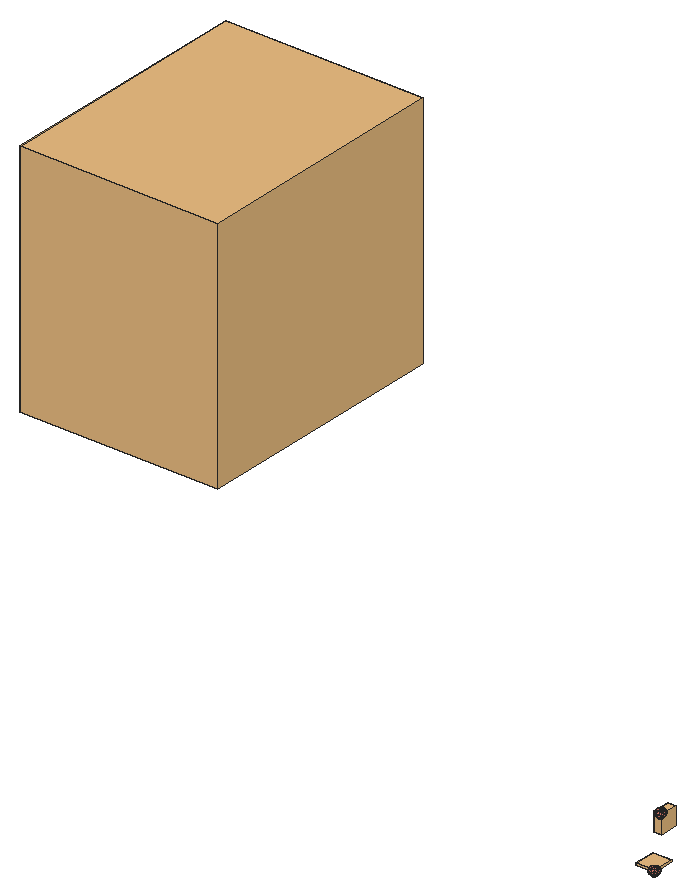
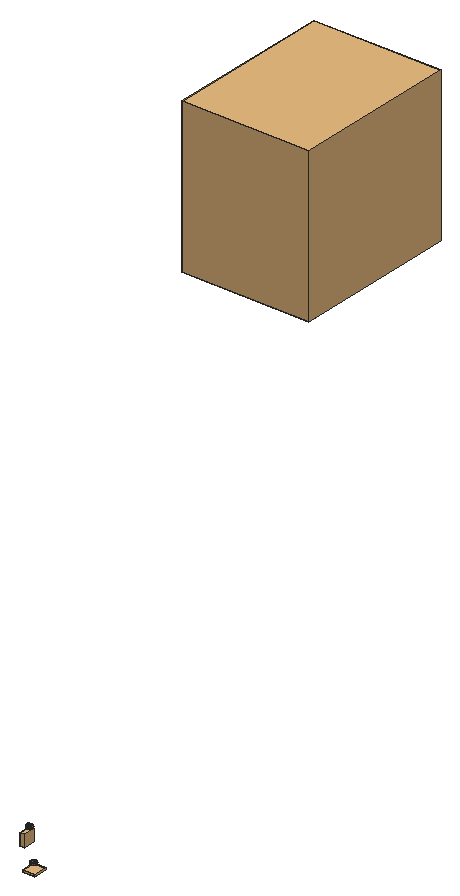
# SketchUp Ruby script. Lengths in inches.
U = 1.inch
M = Sketchup.active_model
def pt(a) = Geom::Point3d.new(a.map { |v| v * U })
def face(e, loops, mat)
  f = e.add_face(loops[0].map { |a| pt(a) })
  loops[1..].each { |l| e.add_face(l.map { |a| pt(a) }).erase! }
  f.material = f.back_material = mat if mat
  f
end
# faces: each face lists its corners as indices into pts; further lists are holes
def faces(e, pts, list, mat = nil) = list.each { |f| face(e, (f[0].is_a?(Array) ? f : [f]).map { |l| l.map { |i| pts[i] } }, mat) }
# xy, xz, yz: faces in a plane at the given z, y or x. An outline is a flat list of corners, or four numbers for a rectangle; further outlines are holes
def ring(l) = l.size == 4 ? [[l[0], l[1]], [l[2], l[1]], [l[2], l[3]], [l[0], l[3]]] : l.each_slice(2).to_a
def flat(e, list, mat, &to3) = list.each { |f| face(e, (f[0].is_a?(Array) ? f : [f]).map { |l| ring(l).map { |u, v| to3.(u, v) } }, mat) }
def xy(e, z, list, mat = nil) = flat(e, list, mat) { |x, y| [x, y, z] }
def xz(e, y, list, mat = nil) = flat(e, list, mat) { |x, z| [x, y, z] }
def yz(e, x, list, mat = nil) = flat(e, list, mat) { |y, z| [x, y, z] }
def lines(e, pts, list) = list.each { |a, b| e.add_line(pt(pts[a]), pt(pts[b])) }
# prism: a flat outline (further loops are holes) pulled along v
def prism(e, loops, v, mat = nil)
  f = face(e, loops, mat); d = Geom::Vector3d.new(v.map { |x| x * U })
  f.pushpull(f.normal.samedirection?(d) ? d.length : -d.length)
end
def box(e, o, s, mat = nil) = prism(e, [[o, [o[0] + s[0], o[1], o[2]], [o[0] + s[0], o[1] + s[1], o[2]], [o[0], o[1] + s[1], o[2]]]], [0, 0, s[2]], mat)
def at(x, y, z, deg = 0) = Geom::Transformation.translation(pt([x, y, z])) * Geom::Transformation.rotation(ORIGIN, Z_AXIS, deg.degrees)
def axes(o, x, y, z) = Geom::Transformation.new([*x, 0, *y, 0, *z, 0, *pt(o).to_a, 1])
def part(name) = M.definitions.add(name)
# library, detail: a bought-in or finely detailed component or shape, given as its bounding box
def library(name, o, s) = part(name).tap { |d| box(d.entities, o, s) }
def detail(e, o, s) = box(e.add_group.entities, o, s)
def put(e, d, t, mat = nil) = e.add_instance(d, t).tap { |i| i.material = mat if mat }
def group(e, t, mat = nil) = e.add_group.tap { |g| g.transformation = t; g.material = mat if mat }.entities
root = M.entities
M.materials.add("green").color = [174, 139, 102]
M.materials.add("vio").color = [206, 114, 100]
c1 = library("Untitled",[0,0,0],[7.78,10.125,9.38])
c2 = part("3DGeom~190_Defintion")
p = [[103.5625,-60.76,-498.22],[-159.65,90.28,-476.73],[101.5,52.12,-500],[335.44,0,-389.29],[150.07,151.03,-458.14],[-75.51,261.6,-404.23],
  [155.72,-157.36,-453.28],[-156.07,-105.24,-473.65],[-378.01,104.24,-325.73],[-280.86,302.07,-242.01],[-280.86,302.07,-242.01],[-65.73,-272.55,-395.81],
  [-373.88,-121.52,-322.17],[236.28,209.48,-383.86],[73.81,362.83,-275.57],[73.81,362.83,-275.57],[243.99,-211.79,-377.22],[-75.51,261.6,-404.23],
  [-280.86,302.07,-242.01],[-108.44,418.95,-93.44],[-75.51,261.6,-404.23],[73.81,362.83,-275.57],[87.16,-366.83,-264.07],[-269.57,-314.71,-232.28],
  [-65.73,-272.55,-395.81],[87.16,-366.83,-264.07],[-269.57,-314.71,-232.28],[344.72,-209.48,-290.42],[430.93,-151.03,-216.13],[344.72,-209.48,-290.42],
  [335.44,0,-389.29],[479.51,-52.12,-174.27],[335.44,0,-389.29],[477.44,60.76,-176.05],[335.44,0,-389.29],[337.02,211.79,-297.06],
  [425.29,157.36,-221],[335.44,0,-389.29],[337.02,211.79,-297.06],[335.44,0,-389.29],[236.28,209.48,-383.86],[248.29,366.83,-125.23],
  [236.28,209.48,-383.86],[248.29,366.83,-125.23],[337.02,211.79,-297.06],[344.72,-209.48,-290.42],[87.16,-366.83,-264.07],[243.99,-211.79,-377.22],
  [-373.88,-121.52,-322.17],[-495.09,90.28,-87.4375],[-378.01,104.24,-325.73],[-378.01,104.24,-325.73],[-410.95,261.6,-14.9375],[-378.01,104.24,-325.73],
  [-410.95,261.6,-14.9375],[-280.86,302.07,-242.01],[-269.57,-314.71,-232.28],[-491.51,-105.24,-84.36],[-373.88,-121.52,-322.17],[-373.88,-121.52,-322.17],
  [401.18,272.55,6.52],[248.29,366.83,-125.23],[344.72,-209.48,-290.42],[261.64,-362.83,-113.72],[87.16,-366.83,-264.07],[261.64,-362.83,-113.72],
  [344.72,-209.48,-290.42],[93.03,423.58,80.16],[248.29,366.83,-125.23],[87.16,-366.83,-264.07],[-93.03,-423.58,-80.16],[-269.57,-314.71,-232.28],
  [87.16,-366.83,-264.07],[-410.95,261.6,-14.9375],[-261.64,362.83,113.72],[-401.18,-272.55,-6.52],[-269.57,-314.71,-232.28],[-269.57,-314.71,-232.28],
  [-401.18,-272.55,-6.52],[491.51,105.23,84.36],[410.95,-261.6,14.9375],[261.64,-362.83,-113.72],[495.09,-90.28,87.44],[248.29,366.83,-125.23],
  [269.57,314.71,232.28],[401.18,272.55,6.52],[248.29,366.83,-125.23],[269.57,314.71,232.28],[108.44,-418.95,93.44],[410.95,-261.6,14.9375],
  [-87.16,366.83,264.07],[-479.51,52.12,174.27],[-430.93,151.03,216.13],[-410.95,261.6,-14.9375],[-477.44,-60.76,176.05],[-248.29,-366.83,125.23],
  [-401.18,-272.55,-6.52],[-410.95,261.6,-14.9375],[-344.72,209.48,290.42],[-410.95,261.6,-14.9375],[-344.72,209.48,290.42],[-261.64,362.83,113.72],
  [-248.29,-366.83,125.23],[-425.29,-157.36,221],[373.88,121.52,322.17],[269.57,314.71,232.28],[410.95,-261.6,14.9375],[280.86,-302.07,242.01],
  [280.86,-302.07,242.01],[65.73,272.55,395.81],[65.73,272.55,395.81],[269.57,314.71,232.28],[378.01,-104.24,325.73],[280.86,-302.07,242.01],
  [-73.81,-362.83,275.57],[-344.72,209.48,290.42],[-243.99,211.79,377.22],[-243.99,211.79,377.22],[-248.29,-366.83,125.23],[-337.02,-211.79,297.06],
  [-337.02,-211.79,297.06],[-335.44,0,389.29],[-344.72,209.48,290.42],[269.57,314.71,232.28],[65.73,272.55,395.81],[156.07,105.24,473.65],
  [269.57,314.71,232.28],[373.88,121.52,322.17],[75.51,-261.6,404.23],[378.01,-104.24,325.73],[75.51,-261.6,404.23],[280.86,-302.07,242.01],
  [-87.16,366.83,264.07],[-243.99,211.79,377.22],[-155.72,157.36,453.28],[-87.16,366.83,264.07],[-236.28,-209.48,383.86],[-337.02,-211.79,297.06],
  [75.51,-261.6,404.23],[-236.28,-209.48,383.86],[-73.81,-362.83,275.57],[-344.72,209.48,290.42],[-335.44,0,389.29],[-337.02,-211.79,297.06],
  [-236.28,-209.48,383.86],[-335.44,0,389.29],[373.88,121.52,322.17],[159.65,-90.28,476.73],[378.01,-104.24,325.73],[373.88,121.52,322.17],
  [378.01,-104.24,325.73],[75.51,-261.6,404.23],[-335.44,0,389.29],[75.51,-261.6,404.23],[-150.07,-151.03,458.14],[-236.28,-209.48,383.86],
  [-236.28,-209.48,383.86],[-335.44,0,389.29],[-101.5,-52.12,500],[-335.44,0,389.29],[-103.5625,60.76,498.22],[-335.44,0,389.29],
  [-335.44,0,389.29],[75.51,-261.6,404.23]]
faces(c2.entities,p,[[0,1,2],[0,2,3],[2,4,3],[2,1,5],[2,5,4],[6,7,0],[6,0,3],[0,7,1],
  [7,8,1],[1,8,9],[1,10,5],[11,12,7],[6,11,7],[7,12,8],[4,13,3],[4,5,14],
  [4,15,13],[16,11,6],[16,6,3],[17,18,19],[20,19,21],[22,23,24],[16,25,11],[11,26,12],
  [27,16,3],[28,29,30],[31,28,32],[33,31,34],[13,35,3],[36,33,37],[38,36,39],[40,21,41],
  [42,43,44],[45,46,47],[48,49,50],[51,49,52],[53,54,55],[56,57,58],[59,57,49],[38,60,36],
  [38,61,60],[62,63,64],[28,65,66],[21,19,67],[21,67,68],[69,70,71],[63,70,72],[18,73,74],
  [18,74,19],[70,75,76],[77,78,57],[36,79,33],[36,60,79],[28,80,81],[31,80,28],[33,79,82],
  [33,82,31],[31,82,80],[83,84,85],[86,67,87],[63,88,70],[89,88,63],[19,74,90],[19,90,67],
  [57,91,49],[49,91,92],[49,92,93],[78,94,57],[57,94,91],[70,95,96],[88,95,70],[97,92,98],
  [99,100,101],[102,103,78],[78,103,94],[60,104,79],[60,105,104],[106,107,88],[82,108,80],[67,90,109],
  [67,110,111],[79,104,112],[79,112,82],[82,112,113],[88,114,95],[107,114,88],[74,115,116],[74,117,90],
  [118,119,103],[114,120,95],[91,94,121],[92,91,121],[94,103,121],[122,92,121],[103,119,121],[123,124,125],
  [126,125,127],[107,128,114],[129,130,131],[132,133,134],[135,134,124],[114,136,137],[138,139,140],[133,141,142],
  [143,144,145],[146,147,148],[149,125,147],[150,147,151],[134,133,152],[153,154,155],[156,154,157],[154,158,159],
  [158,160,161],[160,134,162],[124,134,160],[124,160,125],[147,154,163],[147,158,154],[125,158,147],[125,160,158]],"vio")
c3 = part("3DGeom~191_Defintion")
p = [[58.83,-275.51,-375.83],[-159.55,-167.25,-431.01],[-6.51,0,-500],[191.37,-130.67,-435.58],[-202.64,130.67,-430.45],[148.28,167.25,-435.02],
  [-68.59,275.51,-374.17],[261.44,-309.94,-219.95],[261.44,-309.94,-219.95],[337.97,-226.32,-254.44],[337.97,-226.32,-254.44],[325.42,14.17,-379.3],
  [325.42,14.17,-379.3],[325.42,14.17,-379.3],[263.34,289.68,-253.47],[31.05,381.54,-216.95],[31.05,381.54,-216.95],[263.34,289.68,-253.47],
  [-36.6875,-381.54,-216.07],[-269.84,-289.68,-246.53],[-36.6875,-381.54,-216.07],[-335.18,-14.17,-370.7],[-344.47,226.32,-245.5625],[-267.08,309.94,-213.07],
  [-267.08,309.94,-213.07],[337.97,-226.32,-254.44],[325.42,14.17,-379.3],[415.36,-142.7,-221.95],[415.36,-142.7,-221.95],[325.42,14.17,-379.3],
  [425.06,120.2,-222.07],[325.42,14.17,-379.3],[263.34,289.68,-253.47],[425.06,120.2,-222.07],[206.3,-371.16,-127.71],[-36.6875,-381.54,-216.07],
  [58.83,-275.51,-375.83],[206.3,-371.16,-127.71],[58.83,-275.51,-375.83],[261.44,-309.94,-219.95],[-68.59,275.51,-374.17],[-267.08,309.94,-213.07],
  [-209.55,371.16,-122.29],[-68.59,275.51,-374.17],[31.05,381.54,-216.95],[-430.69,-120.2,-210.9375],[-430.69,-120.2,-210.9375],[-420.99,142.7,-211.06],
  [-335.18,-14.17,-370.7],[-420.99,142.7,-211.06],[261.44,-309.94,-219.95],[337.97,-226.32,-254.44],[394.01,-261.34,-5.125],[394.01,-261.34,-5.125],
  [263.34,289.68,-253.47],[307.83,334.49,-4.01],[263.34,289.68,-253.47],[69.59,420.35,-0.9],[263.34,289.68,-253.47],[307.83,334.49,-4.01],
  [-69.59,-420.35,0.9],[-307.83,-334.49,4.01],[-269.84,-289.68,-246.53],[-269.84,-289.68,-246.53],[-307.83,-334.49,4.01],[-430.69,-120.2,-210.9375],
  [-269.84,-289.68,-246.53],[-344.47,226.32,-245.5625],[-420.99,142.7,-211.06],[-394.01,261.34,5.125],[-267.08,309.94,-213.07],[-344.47,226.32,-245.5625],
  [472.89,-81.48,-131.17],[463.59,159.01,-6.03],[394.01,-261.34,-5.125],[206.3,-371.16,-127.71],[394.01,-261.34,-5.125],[-187.3,393.57,2.4375],
  [187.3,-393.57,-2.4375],[206.3,-371.16,-127.71],[-209.55,371.16,-122.29],[-267.08,309.94,-213.07],[-430.69,-120.2,-210.9375],[-476.14,81.48,-118.83],
  [-420.99,142.7,-211.06],[-420.99,142.7,-211.06],[-307.83,-334.49,4.01],[-463.59,-159.01,6.03],[-430.69,-120.2,-210.9375],[-430.69,-120.2,-210.9375],
  [495.13,-59.08,-6.44],[394.01,-261.34,-5.125],[206.3,-371.16,-127.71],[394.01,-261.34,-5.125],[-394.01,261.34,5.125],[-495.13,59.08,6.44],
  [476.14,-81.48,118.83],[394.01,-261.34,-5.125],[430.69,120.2,210.9375],[269.84,289.68,246.53],[269.84,289.68,246.53],[209.55,-371.16,122.29],
  [267.08,-309.94,213.07],[209.55,-371.16,122.29],[394.01,-261.34,-5.125],[344.47,-226.32,245.5625],[394.01,-261.34,-5.125],[420.99,-142.7,211.06],
  [394.01,-261.34,-5.125],[394.01,-261.34,-5.125],[307.83,334.49,-4.01],[36.6875,381.54,216.07],[269.84,289.68,246.53],[307.83,334.49,-4.01],
  [36.6875,381.54,216.07],[-206.3,371.16,127.71],[36.6875,381.54,216.07],[-31.05,-381.54,216.95],[-394.01,261.34,5.125],[-263.34,-289.68,253.47],
  [-263.34,-289.68,253.47],[-307.83,-334.49,4.01],[-472.89,81.48,131.17],[-415.36,142.7,221.95],[-337.97,226.32,254.44],[-337.97,226.32,254.44],
  [-261.44,309.94,219.95],[-261.44,309.94,219.95],[-206.3,371.16,127.71],[-263.34,-289.68,253.47],[-425.06,-120.2,222.07],[335.18,14.17,370.7],
  [335.18,14.17,370.7],[267.08,-309.94,213.07],[36.6875,381.54,216.07],[-261.44,309.94,219.95],[-325.42,-14.17,379.3],[-325.42,-14.17,379.3],
  [430.69,120.2,210.9375],[159.55,167.25,431.01],[335.18,14.17,370.7],[430.69,120.2,210.9375],[269.84,289.68,246.53],[420.99,-142.7,211.06],
  [202.64,-130.67,430.45],[344.47,-226.32,245.5625],[420.99,-142.7,211.06],[267.08,-309.94,213.07],[68.59,-275.51,374.17],[344.47,-226.32,245.5625],
  [68.59,-275.51,374.17],[267.08,-309.94,213.07],[36.6875,381.54,216.07],[-261.44,309.94,219.95],[-58.83,275.51,375.83],[36.6875,381.54,216.07],
  [-58.83,275.51,375.83],[68.59,-275.51,374.17],[-263.34,-289.68,253.47],[-31.05,-381.54,216.95],[-261.44,309.94,219.95],[-337.97,226.32,254.44],
  [-191.37,130.67,435.58],[-415.36,142.7,221.95],[-325.42,-14.17,379.3],[-415.36,142.7,221.95],[-148.28,-167.25,435.02],[-425.06,-120.2,222.07],
  [-263.34,-289.68,253.47],[-425.06,-120.2,222.07],[344.47,-226.32,245.5625],[68.59,-275.51,374.17],[68.59,-275.51,374.17],[-263.34,-289.68,253.47],
  [6.51,0,500],[68.59,-275.51,374.17]]
faces(c3.entities,p,[[0,1,2],[0,2,3],[1,4,2],[3,2,5],[2,4,6],[2,6,5],[7,0,3],[8,3,9],
  [10,3,11],[3,5,12],[13,5,14],[5,6,15],[5,16,17],[18,19,1],[20,1,0],[19,21,1],
  [1,21,4],[21,22,4],[4,22,23],[4,24,6],[25,26,27],[28,29,30],[31,32,33],[34,35,36],
  [37,38,39],[40,41,42],[43,42,44],[19,45,21],[46,47,48],[21,49,22],[50,51,52],[51,28,53],
  [30,54,55],[56,44,57],[58,57,59],[60,61,62],[60,63,35],[64,65,66],[67,68,69],[70,71,69],
  [28,30,72],[72,30,73],[30,55,73],[28,72,74],[75,50,76],[44,42,77],[44,77,57],[78,60,35],
  [78,35,79],[80,81,69],[82,83,84],[85,83,69],[86,87,88],[87,83,89],[72,90,91],[72,73,90],
  [78,92,93],[77,42,94],[87,95,83],[83,95,69],[90,96,97],[90,98,96],[90,73,98],[73,99,98],
  [73,55,100],[101,78,93],[102,103,104],[105,102,106],[107,105,108],[96,107,109],[110,111,112],[113,57,114],
  [101,60,78],[57,77,115],[57,115,116],[117,61,60],[101,117,60],[115,77,118],[117,119,61],[120,87,121],
  [95,122,69],[122,123,69],[123,124,69],[125,126,69],[127,128,69],[129,130,87],[130,95,87],[130,122,95],
  [96,131,107],[96,98,132],[133,117,101],[134,115,135],[136,122,130],[137,123,122],[138,139,140],[141,142,139],
  [143,144,145],[146,140,144],[147,148,117],[149,150,151],[152,153,154],[142,155,156],[157,158,159],[156,160,161],
  [162,163,164],[162,161,165],[166,167,168],[166,164,169],[170,144,171],[142,156,139],[172,166,173],[156,161,162],
  [140,174,144],[140,139,174],[144,166,175],[139,156,162],[174,164,166],[174,162,164],[144,174,166],[139,162,174]],"vio")
c4 = library("3DGeom~11_Defintion",[-500,-49.41,-434.02],[1000,98.82,868.04])
c5 = part("3DGeom~12_Defintion")
p = [[-473.91,-42.88,-428.57],[-493.27,-23.3125,-425.27],[-480.23,-29.84,-434.02],[-473.91,-42.88,-428.57],[-480.23,-29.84,-434.02],[-475.54,-36.36,-433.07],
  [-493.27,-23.3125,-425.27],[-486.72,-25.0625,-431.16],[-480.23,-29.84,-434.02],[-480.63,-49.41,-414.38],[-493.27,-23.3125,-425.27],[-473.91,-42.88,-428.57],
  [-480.63,-49.41,-414.38],[-473.91,-42.88,-428.57],[-475.77,-47.66,-421.73],[-493.68,-42.88,-405.63],[-493.27,-23.3125,-425.27],[-480.63,-49.41,-414.38],
  [-500,-29.84,-411.07],[-493.27,-23.3125,-425.27],[-493.68,-42.88,-405.63],[-493.27,-23.3125,-425.27],[-498.13,-25.0625,-417.92],[-493.68,-42.88,-405.63],
  [-480.63,-49.41,-414.38],[-487.1875,-47.66,-408.48],[-493.68,-42.88,-405.63],[-498.37,-36.36,-406.58],[489.39,27.6,421.47],[498.07,5.37,408.95],
  [500,12.78,407.52],[489.39,27.6,421.47],[500,12.78,407.52],[498.875,20.1875,409.65],[489.39,27.6,421.47],[493.59,-0.05,413.55],
  [498.07,5.37,408.95],[489.39,27.6,421.47],[498.875,20.1875,409.65],[494.99,25.61,414.75],[489.39,27.6,421.47],[487.78,-2.04,420.08],
  [493.59,-0.05,413.55],[489.39,27.6,421.47],[482.18,-0.05,426.79],[487.78,-2.04,420.08],[489.39,27.6,421.47],[478.3,5.37,431.9],
  [482.18,-0.05,426.79],[489.39,27.6,421.47],[477.17,12.78,434.02],[478.3,5.37,431.9],[489.39,27.6,421.47],[479.1,20.1875,432.59],
  [477.17,12.78,434.02],[489.39,27.6,421.47],[483.58,25.61,428],[479.1,20.1875,432.59]]
faces(c5.entities,p,[[0,1,2],[3,4,5],[6,7,8],[9,10,11],[12,13,14],[15,16,17],[18,19,20],[21,18,22],
  [23,24,25],[18,26,27],[28,29,30],[31,32,33],[34,35,36],[37,38,39],[40,41,42],[43,44,45],
  [46,47,48],[49,50,51],[52,53,54],[55,56,57]],"green")
c6 = library("3DGeom~13_Defintion",[-468.3,-500,-197.66],[936.6,1000,395.32])
c7 = part("3DGeom~14_Defintion")
p = [[-455.16,-492.22,-183.4],[-446.73,-497.16,-180.84],[-439.77,-500,-173.64],[-436.83,-497.09,-153.74],[-455.16,-492.22,-183.4],[-439.77,-500,-173.64],
  [-449.28,-486.4,-143.61],[-455.16,-492.22,-183.4],[-436.83,-497.09,-153.74],[-467.61,-481.53,-173.27],[-455.16,-492.22,-183.4],[-464.67,-478.62,-153.38],
  [-455.16,-492.22,-183.4],[-467.61,-481.53,-173.27],[-462.81,-486.5,-180.63],[-464.67,-478.62,-153.38],[-455.16,-492.22,-183.4],[-449.28,-486.4,-143.61],
  [-436.83,-497.09,-153.74],[-439.77,-500,-173.64],[-436.15,-499.97,-163.72],[-467.61,-481.53,-173.27],[-464.67,-478.62,-153.38],[-468.3,-478.65,-163.3],
  [-449.28,-486.4,-143.61],[-436.83,-497.09,-153.74],[-441.64,-492.12,-146.38],[-464.67,-478.62,-153.38],[-449.28,-486.4,-143.61],[-457.71,-481.46,-146.17],
  [456.2,493.0625,159.13],[456.82,479.16,194.97],[464.16,476.9375,187.85],[456.2,493.0625,159.13],[464.16,476.9375,187.85],[468.3,477.81,178.18],
  [456.2,493.0625,159.13],[468.3,477.81,178.18],[468.13,481.53,168.58],[456.2,493.0625,159.13],[448.25,483.875,197.66],[456.82,479.16,194.97],
  [456.2,493.0625,159.13],[468.13,481.53,168.58],[463.7,487.12,161.6],[456.2,493.0625,159.13],[440.74,489.82,195.18],[448.25,483.875,197.66],
  [456.2,493.0625,159.13],[436.3125,495.41,188.21],[440.74,489.82,195.18],[456.2,493.0625,159.13],[436.15,499.13,178.6],[436.3125,495.41,188.21],
  [456.2,493.0625,159.13],[440.29,500,168.94],[436.15,499.13,178.6],[456.2,493.0625,159.13],[447.63,497.78,161.8125],[440.29,500,168.94]]
faces(c7.entities,p,[[0,1,2],[3,4,5],[6,7,8],[9,10,11],[12,13,14],[15,16,17],[18,19,20],[21,22,23],
  [24,25,26],[27,28,29],[30,31,32],[33,34,35],[36,37,38],[39,40,41],[42,43,44],[45,46,47],
  [48,49,50],[51,52,53],[54,55,56],[57,58,59]],"green")
put(root,c1,at(12.99,12.95,61.14))
g1 = group(root,at(15.3125,38.42,26.21))
put(g1,c2,axes([2.9,-0.75,9.71],[0,0.00038,0],[0,0,-0.00038],[-0.00038,0,0]),"vio")
g2 = group(root,at(15.3125,38.42,26.21))
put(g2,c3,axes([3.03,-0.6,11.73],[0,0.00039,0],[0,0,-0.00039],[-0.00039,0,0]),"vio")
g3 = group(root,at(15.3125,38.42,26.21))
put(g3,c4,axes([2.51,-0.3,9.67],[0,0.00085,0],[0,0,-0.00085],[-0.00085,0,0]),"green")
put(g3,c5,axes([2.51,-0.3,9.67],[0,0.00085,0],[0,0,-0.00085],[-0.00085,0,0]),"green")
g4 = group(root,at(15.3125,38.42,26.21))
put(g4,c6,axes([2.91,-0.25,11.34],[0,0.00073,0],[0,0,-0.00073],[-0.00073,0,0]),"green")
put(g4,c7,axes([2.91,-0.25,11.34],[0,0.00073,0],[0,0,-0.00073],[-0.00073,0,0]),"green")
